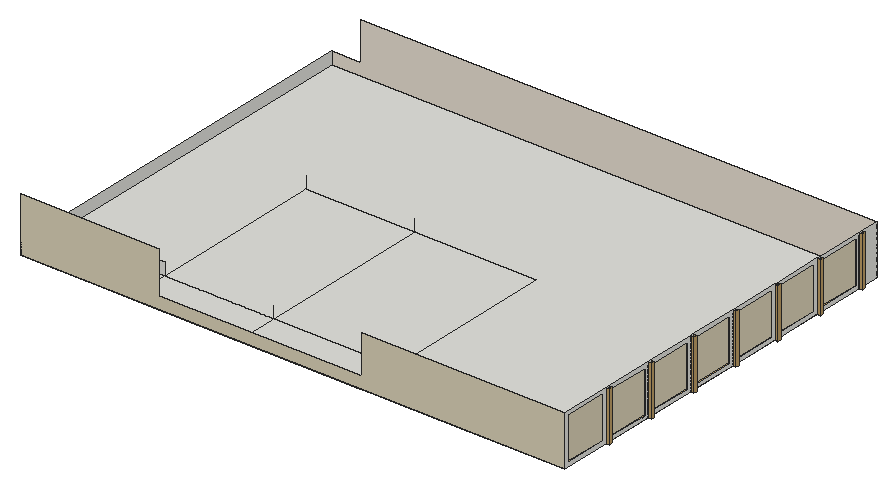
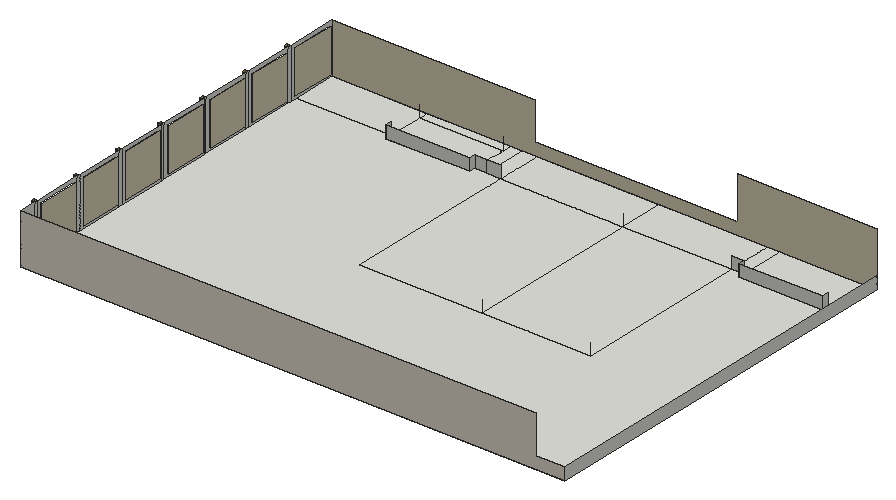
# SketchUp Ruby script. Lengths in inches.
U = 1.inch
M = Sketchup.active_model
def pt(a) = Geom::Point3d.new(a.map { |v| v * U })
def face(e, loops, mat)
  f = e.add_face(loops[0].map { |a| pt(a) })
  loops[1..].each { |l| e.add_face(l.map { |a| pt(a) }).erase! }
  f.material = f.back_material = mat if mat
  f
end
# faces: each face lists its corners as indices into pts; further lists are holes
def faces(e, pts, list, mat = nil) = list.each { |f| face(e, (f[0].is_a?(Array) ? f : [f]).map { |l| l.map { |i| pts[i] } }, mat) }
# xy, xz, yz: faces in a plane at the given z, y or x. An outline is a flat list of corners, or four numbers for a rectangle; further outlines are holes
def ring(l) = l.size == 4 ? [[l[0], l[1]], [l[2], l[1]], [l[2], l[3]], [l[0], l[3]]] : l.each_slice(2).to_a
def flat(e, list, mat, &to3) = list.each { |f| face(e, (f[0].is_a?(Array) ? f : [f]).map { |l| ring(l).map { |u, v| to3.(u, v) } }, mat) }
def xy(e, z, list, mat = nil) = flat(e, list, mat) { |x, y| [x, y, z] }
def xz(e, y, list, mat = nil) = flat(e, list, mat) { |x, z| [x, y, z] }
def yz(e, x, list, mat = nil) = flat(e, list, mat) { |y, z| [x, y, z] }
def lines(e, pts, list) = list.each { |a, b| e.add_line(pt(pts[a]), pt(pts[b])) }
# prism: a flat outline (further loops are holes) pulled along v
def prism(e, loops, v, mat = nil)
  f = face(e, loops, mat); d = Geom::Vector3d.new(v.map { |x| x * U })
  f.pushpull(f.normal.samedirection?(d) ? d.length : -d.length)
end
def box(e, o, s, mat = nil) = prism(e, [[o, [o[0] + s[0], o[1], o[2]], [o[0] + s[0], o[1] + s[1], o[2]], [o[0], o[1] + s[1], o[2]]]], [0, 0, s[2]], mat)
def at(x, y, z, deg = 0) = Geom::Transformation.translation(pt([x, y, z])) * Geom::Transformation.rotation(ORIGIN, Z_AXIS, deg.degrees)
def axes(o, x, y, z) = Geom::Transformation.new([*x, 0, *y, 0, *z, 0, *pt(o).to_a, 1])
def part(name) = M.definitions.add(name)
# library, detail: a bought-in or finely detailed component or shape, given as its bounding box
def library(name, o, s) = part(name).tap { |d| box(d.entities, o, s) }
def detail(e, o, s) = box(e.add_group.entities, o, s)
def put(e, d, t, mat = nil) = e.add_instance(d, t).tap { |i| i.material = mat if mat }
def group(e, t, mat = nil) = e.add_group.tap { |g| g.transformation = t; g.material = mat if mat }.entities
root = M.entities
M.materials.add("Generic").color = [191, 159, 103]
M.materials.add("Generic\#3").color = [218, 209, 183]
M.materials.add("Generic\#5").color = [230, 221, 208]
xy(root,-21.1875,[[4.1875,5.75,25.82,83.8125],[25.82,5.75,171.85,94.5625],[171.85,5.75,193.48,83.8125],[193.48,5.75,382.78,83.8125],[382.78,5.75,596.08,83.8125],
  [596.08,5.75,620.08,83.8125],[620.08,5.75,641.71,83.8125],[641.71,5.75,787.75,20.625],[787.75,5.75,952.875,83.8125],[641.71,20.625,787.75,94.5625],
  [4.1875,83.8125,4.1875,683.8125,952.875,683.8125,952.875,83.8125,787.75,83.8125,787.75,94.5625,641.71,94.5625,641.71,83.8125,596.08,83.8125,596.08,391.4375,193.48,391.4375,193.48,83.8125,171.85,83.8125,171.85,94.5625,25.82,94.5625,25.82,83.8125],[193.48,83.8125,382.78,391.4375],[382.78,83.8125,596.08,391.4375],[952.875,95.32,958.625,100.94],[952.875,187.19,958.625,192.82],
  [952.875,279.07,958.625,284.69],[952.875,370.94,958.625,376.57],[952.875,462.82,958.625,468.44],[952.875,554.69,958.625,560.32],[952.875,646.57,958.625,652.19]])
xy(root,-14.89,[[950.0625,12.05,952.875,89.02],[950.0625,107.24,952.875,180.9],[950.0625,199.12,952.875,272.77],[950.0625,290.99,952.875,364.65],[950.0625,382.87,952.875,456.52],
  [950.0625,474.74,952.875,548.4],[950.0625,566.62,952.875,640.27]],"Generic")
xz(root,5.75,[[4.1875,-21.1875,952.875,-21.1875,952.875,66.1875,599.47,66.1875,599.47,0,245.8125,0,245.8125,74,4.1875,74]],"Generic\#3")
xz(root,12.05,[[950.0625,-14.89,952.875,59.89]],"Generic")
xz(root,83.8125,[[171.85,-21.1875,193.48,0],[596.08,-21.1875,620.08,0],[620.08,-21.1875,641.71,0]])
xz(root,89.02,[[950.0625,-14.89,952.875,59.89]],"Generic")
xz(root,94.5625,[[25.82,-21.1875,171.85,0],[641.71,-21.1875,787.75,0]])
xz(root,95.32,[[952.875,-21.1875,958.625,66.1875]],"Generic")
xz(root,100.94,[[952.875,-21.1875,958.625,66.1875]],"Generic")
xz(root,107.24,[[950.0625,-14.89,952.875,59.89]],"Generic")
xz(root,180.9,[[950.0625,-14.89,952.875,59.89]],"Generic")
xz(root,187.19,[[952.875,-21.1875,958.625,66.1875]],"Generic")
xz(root,192.82,[[952.875,-21.1875,958.625,66.1875]],"Generic")
xz(root,199.12,[[950.0625,-14.89,952.875,59.89]],"Generic")
xz(root,272.77,[[950.0625,-14.89,952.875,59.89]],"Generic")
xz(root,279.07,[[952.875,-21.1875,958.625,66.1875]],"Generic")
xz(root,284.69,[[952.875,-21.1875,958.625,66.1875]],"Generic")
xz(root,290.99,[[950.0625,-14.89,952.875,59.89]],"Generic")
xz(root,364.65,[[950.0625,-14.89,952.875,59.89]],"Generic")
xz(root,370.94,[[952.875,-21.1875,958.625,66.1875]],"Generic")
xz(root,376.57,[[952.875,-21.1875,958.625,66.1875]],"Generic")
xz(root,382.87,[[950.0625,-14.89,952.875,59.89]],"Generic")
xz(root,456.52,[[950.0625,-14.89,952.875,59.89]],"Generic")
xz(root,462.82,[[952.875,-21.1875,958.625,66.1875]],"Generic")
xz(root,468.44,[[952.875,-21.1875,958.625,66.1875]],"Generic")
xz(root,474.74,[[950.0625,-14.89,952.875,59.89]],"Generic")
xz(root,548.4,[[950.0625,-14.89,952.875,59.89]],"Generic")
xz(root,554.69,[[952.875,-21.1875,958.625,66.1875]],"Generic")
xz(root,560.32,[[952.875,-21.1875,958.625,66.1875]],"Generic")
xz(root,566.62,[[950.0625,-14.89,952.875,59.89]],"Generic")
xz(root,640.27,[[950.0625,-14.89,952.875,59.89]],"Generic")
xz(root,646.57,[[952.875,-21.1875,958.625,66.1875]],"Generic")
xz(root,652.19,[[952.875,-21.1875,958.625,66.1875]],"Generic")
xz(root,683.8125,[[4.1875,-21.1875,4.1875,0,55.33,0,55.33,66.1875,952.875,66.1875,952.875,-21.1875]],"Generic\#5")
yz(root,4.1875,[[5.75,-21.1875,683.8125,0]])
yz(root,25.82,[[83.8125,-21.1875,94.5625,0]])
yz(root,171.85,[[83.8125,-21.1875,94.5625,0]])
yz(root,641.71,[[83.8125,-21.1875,94.5625,0]])
yz(root,787.75,[[83.8125,-21.1875,94.5625,0]])
yz(root,950.0625,[[12.05,-14.89,89.02,59.89],[107.24,-14.89,180.9,59.89],[199.12,-14.89,272.77,59.89],[290.99,-14.89,364.65,59.89],[382.87,-14.89,456.52,59.89],
  [474.74,-14.89,548.4,59.89],[566.62,-14.89,640.27,59.89]],"Generic\#3")
yz(root,952.875,[[[5.75,-21.1875,95.32,66.1875],[12.05,-14.89,89.02,59.89]],[95.32,-21.1875,100.94,66.1875],[[100.94,-21.1875,187.19,66.1875],[107.24,-14.89,180.9,59.89]],[187.19,-21.1875,192.82,66.1875],[[192.82,-21.1875,279.07,66.1875],[199.12,-14.89,272.77,59.89]],
  [279.07,-21.1875,284.69,66.1875],[[284.69,-21.1875,370.94,66.1875],[290.99,-14.89,364.65,59.89]],[370.94,-21.1875,376.57,66.1875],[[376.57,-21.1875,462.82,66.1875],[382.87,-14.89,456.52,59.89]],[462.82,-21.1875,468.44,66.1875],
  [[468.44,-21.1875,554.69,66.1875],[474.74,-14.89,548.4,59.89]],[554.69,-21.1875,560.32,66.1875],[[560.32,-21.1875,646.57,66.1875],[566.62,-14.89,640.27,59.89]],[646.57,-21.1875,652.19,66.1875],[652.19,-21.1875,683.8125,66.1875]])
yz(root,958.625,[[95.32,-21.1875,100.94,66.1875],[187.19,-21.1875,192.82,66.1875],[279.07,-21.1875,284.69,66.1875],[370.94,-21.1875,376.57,66.1875],[462.82,-21.1875,468.44,66.1875],
  [554.69,-21.1875,560.32,66.1875],[646.57,-21.1875,652.19,66.1875]],"Generic")
p = [[382.78,391.4375,0],[382.78,391.4375,-21.1875],[193.48,391.4375,0],[193.48,391.4375,-21.1875],[382.78,83.8125,0],[382.78,83.8125,-21.1875],
  [641.71,20.625,0],[641.71,20.625,-21.1875],[787.75,20.625,0],[787.75,20.625,-21.1875]]
lines(root,p,[[0,1],[2,3],[4,5],[6,7],[8,9]])
